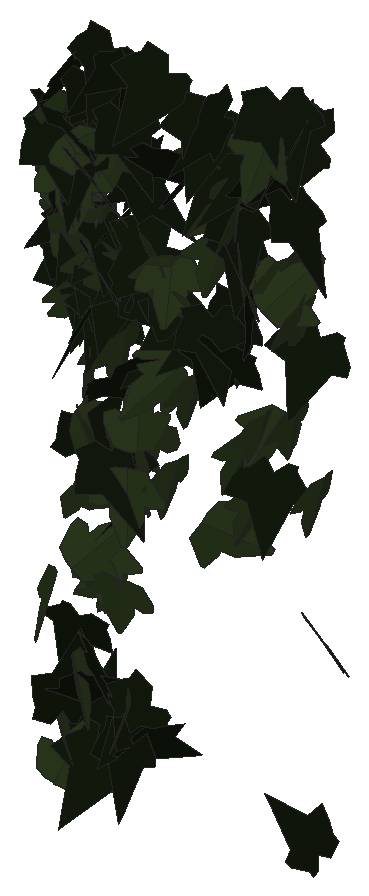
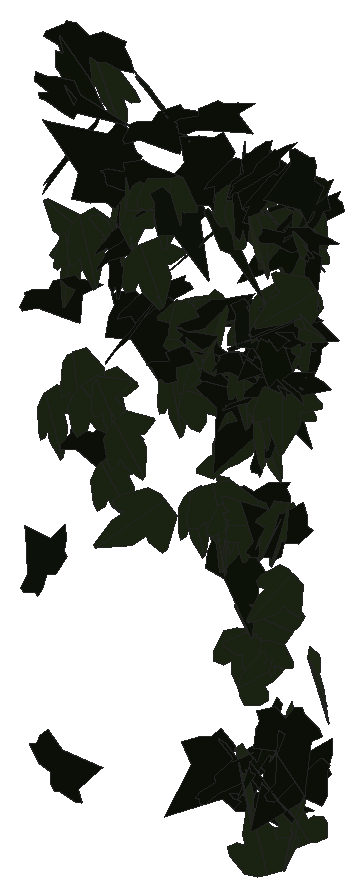
# SketchUp Ruby script. Lengths in inches.
U = 1.inch
M = Sketchup.active_model
def pt(a) = Geom::Point3d.new(a.map { |v| v * U })
def face(e, loops, mat)
  f = e.add_face(loops[0].map { |a| pt(a) })
  loops[1..].each { |l| e.add_face(l.map { |a| pt(a) }).erase! }
  f.material = f.back_material = mat if mat
  f
end
# faces: each face lists its corners as indices into pts; further lists are holes
def faces(e, pts, list, mat = nil) = list.each { |f| face(e, (f[0].is_a?(Array) ? f : [f]).map { |l| l.map { |i| pts[i] } }, mat) }
# xy, xz, yz: faces in a plane at the given z, y or x. An outline is a flat list of corners, or four numbers for a rectangle; further outlines are holes
def ring(l) = l.size == 4 ? [[l[0], l[1]], [l[2], l[1]], [l[2], l[3]], [l[0], l[3]]] : l.each_slice(2).to_a
def flat(e, list, mat, &to3) = list.each { |f| face(e, (f[0].is_a?(Array) ? f : [f]).map { |l| ring(l).map { |u, v| to3.(u, v) } }, mat) }
def xy(e, z, list, mat = nil) = flat(e, list, mat) { |x, y| [x, y, z] }
def xz(e, y, list, mat = nil) = flat(e, list, mat) { |x, z| [x, y, z] }
def yz(e, x, list, mat = nil) = flat(e, list, mat) { |y, z| [x, y, z] }
def lines(e, pts, list) = list.each { |a, b| e.add_line(pt(pts[a]), pt(pts[b])) }
# prism: a flat outline (further loops are holes) pulled along v
def prism(e, loops, v, mat = nil)
  f = face(e, loops, mat); d = Geom::Vector3d.new(v.map { |x| x * U })
  f.pushpull(f.normal.samedirection?(d) ? d.length : -d.length)
end
def box(e, o, s, mat = nil) = prism(e, [[o, [o[0] + s[0], o[1], o[2]], [o[0] + s[0], o[1] + s[1], o[2]], [o[0], o[1] + s[1], o[2]]]], [0, 0, s[2]], mat)
def at(x, y, z, deg = 0) = Geom::Transformation.translation(pt([x, y, z])) * Geom::Transformation.rotation(ORIGIN, Z_AXIS, deg.degrees)
def axes(o, x, y, z) = Geom::Transformation.new([*x, 0, *y, 0, *z, 0, *pt(o).to_a, 1])
def part(name) = M.definitions.add(name)
# library, detail: a bought-in or finely detailed component or shape, given as its bounding box
def library(name, o, s) = part(name).tap { |d| box(d.entities, o, s) }
def detail(e, o, s) = box(e.add_group.entities, o, s)
def put(e, d, t, mat = nil) = e.add_instance(d, t).tap { |i| i.material = mat if mat }
def group(e, t, mat = nil) = e.add_group.tap { |g| g.transformation = t; g.material = mat if mat }.entities
root = M.entities
M.materials.add("efeu1").color = [18, 25, 13]
M.materials.add("efeu2").color = [43, 57, 29]
c1 = part("ivyleaf_9")
p = [[1.54,2.16,1.25],[1.36,2.04,1.19],[-0.21,0.99,0.68],[-0.71,1.11,0.82],[-0.85,0.86,0.67],[-0.8,0.17,0.21],
  [-0.9,-0.01,0.1],[-0.67,-0.16,-0.02],[-0.08,-0.08,-0.05],[-0.03,-0.6,-0.4],[0.65,-0.88,-0.66],[0.83,-0.6,-0.49],
  [1.29,-0.42,-0.43],[1.8125,-0.07,-0.26],[1.21,0.44,0.15]]
faces(c1.entities,p,[[0,1,2,3,4,5,6,7,8,9,10,11,12,13,14]],"efeu1")
c2 = part("ivyleaf_10")
p = [[0,0.5,-0.03],[-0.0625,2.02,-0.43],[-0.19,2.01,-0.46],[-0.54,1.05,-0.29],[-0.52,0.625,-0.18],[-0.83,0.76,-0.28],
  [-1.16,0.64,-0.33],[-1.15,0.33,-0.24],[-0.77,-0.39,0.02],[-0.3,-0.51,0.16],[0.04,-0.48,0.23],[-0.02,2.01,-0.4375],
  [-0.06,2.01,-0.43],[0.04,-0.49,0.23],[0.67,-0.49,0.14],[1.38,0.36,-0.2],[1.375,0.51,-0.24],[0.81,0.65,-0.19],
  [0.62,0.59,-0.15],[0.6,1.09,-0.28],[0.5,1.23,-0.31]]
faces(c2.entities,p,[[0,1,2,3,4,5,6,7,8,9,10],[11,12,0,13,14,15,16,17,18,19,20]],"efeu2")
put(root,c1,axes([507.83,132.65,201.51],[0.08823,-0.14914,0.79199],[-0.21475,0.73614,0.17212],[-0.81009,-0.21139,0.04063]))
put(root,c1,axes([507.59,132.8,204.79],[-0.22478,0.50304,-0.56535],[-0.28414,0.47763,0.56442],[0.74774,0.33272,0.04453]))
put(root,c2,axes([507.55,132.72,188.94],[0.5578,-0.63656,0.09202],[0.06028,-0.06866,-0.85253],[0.69148,0.51949,0.00008]))
put(root,c1,axes([507.84,133.64,187.58],[0.3913,0.28613,-0.55356],[-0.43338,-0.35012,-0.47981],[-0.48799,0.54037,-0.01777]))
put(root,c2,axes([507.55,133.21,203.85],[0.11682,-0.66008,0.56389],[0.20973,-0.53066,-0.66464],[0.84243,0.22365,0.08727]))
put(root,c2,axes([508.34,133.24,200.28],[0.14149,0.1442,0.84892],[-0.89486,-0.00054,0.13841],[0.02527,-0.82671,0.14798]))
put(root,c1,axes([507.72,133.79,203.49],[-0.62241,-0.5033,-0.11717],[0.16276,-0.00276,-0.7889],[0.5327,-0.58721,0.10414]))
put(root,c2,axes([507.35,133.46,201.4],[0.29609,0.231,0.69601],[0.33312,0.60701,-0.34931],[-0.68825,0.39318,0.13036]))
put(root,c2,axes([507.83,133.82,198.22],[-0.40944,-0.70221,-0.07221],[0.04586,0.05597,-0.82985],[0.7607,-0.38133,0.01116]))
put(root,c1,axes([508.04,133.86,200.75],[-0.03628,-0.00307,-0.74142],[-0.02421,-0.71334,0.0043],[-0.76957,0.02259,0.03482]))
put(root,c2,axes([507.92,132.95,184.39],[-0.48542,0.61504,0.36711],[-0.21163,0.29393,-0.79211],[-0.73605,-0.49013,-0.01435]))
put(root,c1,axes([507.71,134.01,198.78],[-0.35915,-0.66076,-0.26235],[0.15194,0.21138,-0.76872],[0.74859,-0.35991,0.03016]))
put(root,c1,axes([508.11,134.05,199.85],[-0.44002,0.41627,-0.41612],[0.29026,-0.29669,-0.60563],[-0.55191,-0.48792,0.01325]))
put(root,c1,axes([507.94,132.85,185.15],[-0.29979,-0.38919,0.71445],[0.55362,0.46502,0.4894],[-0.64856,0.57684,0.08751]))
put(root,c1,axes([507.4375,133.03,204.11],[0.52831,-0.60031,0.08765],[0.16106,0.01421,-0.79498],[0.63457,0.49618,0.12881]))
put(root,c2,axes([507.87,133.06,199.88],[-0.73165,0.39673,-0.31358],[0.26626,-0.16665,-0.83209],[-0.42992,-0.77838,0.01832]))
put(root,c2,axes([508.18,133.49,197.84],[-0.61701,-0.45043,-0.12896],[0.10779,0.07369,-0.7566],[0.49291,-0.57994,0.00403]))
put(root,c1,axes([507.875,132.69,203.6],[0.05112,-0.8027,-0.32007],[-0.03615,0.30627,-0.83612],[0.92774,0.05617,-0.01494]))
put(root,c2,axes([508.23,133.42,193.97],[-0.59195,0.42254,0.1104],[-0.09381,0.06119,-0.71973],[-0.46107,-0.55492,0.0047]))
put(root,c1,axes([508.02,132.7,185.82],[0.6078,0.5937,0.15759],[0.10716,0.11474,-0.85074],[-0.65302,0.57142,0.00708]))
put(root,c2,axes([508.0625,133.46,191.89],[-0.28471,-0.36404,-0.5651],[0.33352,0.44715,-0.46738],[0.62267,-0.40596,-0.00804]))
put(root,c2,axes([508.21,133.37,194.08],[-0.04122,0.6181,0.34369],[-0.01625,0.33016,-0.64403],[-0.7568,-0.04075,-0.00489]))
put(root,c1,axes([508.43,133.56,200.625],[-0.65499,-0.43701,-0.09011],[0.07869,0.04708,-0.77741],[0.47468,-0.61082,0.00455]))
put(root,c1,axes([508.15,133.42,193.22],[-0.24418,-0.12481,0.67841],[0.63607,0.28081,0.26817],[-0.33152,0.6307,0.01486]))
put(root,c1,axes([507.96,133.28,199.95],[-0.14606,-0.25315,-0.77029],[0.35961,0.66163,-0.29841],[0.76504,-0.35933,-0.00679]))
put(root,c2,axes([508.1,132.52,183.33],[0.6501,0.27358,-0.33388],[0.31047,0.14327,0.68756],[0.33334,-0.66698,0.01075]))
put(root,c2,axes([507.84,132.91,200.04],[-0.00218,-0.10095,0.80218],[0.78223,0.28117,0.04024],[-0.30651,0.71826,0.097]))
put(root,c1,axes([508.48,133.75,199.83],[-0.53829,-0.51327,-0.22019],[0.22001,0.09562,-0.73983],[0.55782,-0.53302,0.07932]))
put(root,c2,axes([508.6,134.29,188.84],[-0.1192,0.12374,0.75106],[0.06288,-0.72653,0.13872],[0.78881,0.07662,0.10243]))
put(root,c1,axes([508.27,133.57,205],[0.36472,-0.6805,-0.43662],[-0.16234,0.4076,-0.77087],[0.79206,0.39689,0.04306]))
put(root,c1,axes([508.37,133.1,203.06],[-0.60944,-0.31216,-0.57338],[0.65229,-0.04204,-0.61816],[0.20668,-0.7878,0.26018]))
put(root,c1,axes([508.43,134.38,205.51],[-0.14976,-0.77891,0.2669],[-0.03446,-0.26512,-0.79303],[0.82265,-0.15291,0.01537]))
put(root,c1,axes([508.8,132.95,197.97],[-0.45384,0.48819,-0.44189],[0.29717,-0.32377,-0.6699],[-0.63265,-0.50229,0.00232]))
put(root,c1,axes([508.74,133.16,184.51],[-0.69852,0.44966,0.1023],[0.08168,-0.06353,0.81919],[0.49036,0.65112,0.00928]))
put(root,c1,axes([508.59,134.28,199.99],[-0.43553,-0.61017,0.31763],[0.03986,-0.39769,-0.70932],[0.68674,-0.36388,0.24261]))
put(root,c2,axes([508.6875,133.54,200.6875],[-0.02906,-0.81664,0.1158],[0.06027,-0.11295,-0.84755],[0.88809,-0.01905,0.06131]))
put(root,c2,axes([508.66,133.66,196.73],[0.25168,-0.80206,0.1969],[0.04548,-0.19207,-0.8405],[0.82462,0.25538,-0.01374]))
put(root,c2,axes([508.43,132.58,202.53],[0.87773,0.24491,0.12471],[0.12004,0.04671,-0.88267],[-0.26893,0.82019,0.01304]))
put(root,c1,axes([509.01,133.5625,200.31],[-0.36581,0.7294,-0.16348],[0.07341,-0.14174,-0.83637],[-0.80249,-0.34546,-0.00199]))
put(root,c2,axes([508.39,132.72,203.12],[0.33206,0.63205,0.41507],[0.20873,0.34965,-0.73074],[-0.77986,0.36271,-0.01885]))
put(root,c2,axes([508.75,133.92,203.34],[0.34835,-0.66525,0.07882],[0.0303,-0.07063,-0.76887],[0.72248,0.32372,-0.00577]))
put(root,c1,axes([508.875,133.74,198.85],[-0.79284,-0.23796,-0.24781],[0.26839,0.00287,-0.79921],[0.24545,-0.7718,0.07344]))
put(root,c1,axes([508.32,132.69,202.84],[0.84414,-0.26691,-0.04166],[-0.0398,0.01603,-0.85895],[0.28876,0.78247,0.00338]))
put(root,c2,axes([508.66,132.62,186.73],[-0.32703,0.74213,-0.16966],[0.06738,-0.15074,-0.83359],[-0.81787,-0.30916,-0.00084]))
put(root,c1,axes([508.39,133.95,196.16],[0.1022,-0.23603,0.65467],[0.22483,-0.59416,-0.26424],[0.69038,0.22844,-0.01086]))
put(root,c2,axes([508.72,133.58,182.75],[-0.56267,-0.52934,0.14175],[0.10232,0.09812,0.77253],[-0.53836,0.57189,-0.00134]))
put(root,c1,axes([508.71,133.04,186.95],[0.68181,-0.21049,-0.48764],[-0.45179,0.22105,-0.68895],[0.32249,0.75467,0.06579]))
put(root,c2,axes([508.62,133.79,189.76],[0.73936,0.30162,0.12368],[0.1156,0.052,-0.778],[-0.33052,0.69289,0.00455]))
put(root,c1,axes([508.93,134.1,205.1875],[-0.03426,-0.15436,-0.7374],[0.29574,-0.65979,0.13664],[-0.72576,-0.26157,0.09049]))
put(root,c2,axes([508.55,132.95,190.06],[0.37922,0.28564,-0.68694],[0.5192,0.4538,0.46987],[0.57835,-0.59468,0.0286]))
put(root,c2,axes([508.76,132.9375,196.57],[-0.15176,0.31577,-0.70998],[0.25853,-0.63961,-0.35892],[-0.7701,-0.27695,0.01942]))
put(root,c1,axes([508.96,133.86,197.78],[-0.39507,-0.66279,0.20863],[0.11374,-0.27748,-0.75373],[0.73918,-0.31154,0.22748]))
put(root,c2,axes([509.25,132.99,199.7],[-0.69264,-0.49041,0.01584],[-0.01025,-0.01266,-0.83963],[0.52979,-0.64139,0.00446]))
put(root,c1,axes([508.96,134.21,203.55],[0.03827,0.31837,0.73957],[-0.10903,-0.70398,0.33301],[0.83437,-0.1066,0.00959]))
put(root,c2,axes([509.07,134.43,203.58],[-0.05981,-0.18416,-0.78009],[0.0303,-0.752,0.18986],[-0.8336,-0.01412,0.06287]))
put(root,c1,axes([508.89,133.66,200.39],[0.00314,-0.7575,0.31667],[0.12135,-0.31277,-0.74936],[0.81201,0.04967,0.11077]))
put(root,c1,axes([509.44,132.95,184.17],[-0.78406,-0.43411,-0.05905],[0.10459,-0.05201,-0.87424],[0.46112,-0.72634,0.0979]))
put(root,c1,axes([509.27,133.72,199.02],[-0.40992,-0.71059,-0.07124],[0.03052,0.06257,-0.83781],[0.77039,-0.38058,-0.00472]))
put(root,c1,axes([508.9,133.125,199.51],[0.1803,-0.46852,0.59657],[0.30705,-0.50244,-0.51284],[0.73862,0.32323,0.06756]))
put(root,c2,axes([509.63,133.26,189.32],[-0.81636,-0.16825,0.13142],[-0.13501,-0.01997,-0.80533],[0.1828,-0.76612,-0.00786]))
put(root,c2,axes([509.02,134,193.7],[-0.31907,0.09238,-0.68974],[0.67749,-0.21538,-0.32182],[-0.25296,-0.69335,0.00807]))
put(root,c1,axes([509.98,133.21,192.07],[-0.18307,0.81913,0.11633],[-0.06771,0.10111,-0.86892],[-0.8903,-0.17613,0.04217]))
put(root,c2,axes([509.87,133.15,203.66],[-0.61061,-0.49609,0.29463],[-0.13166,-0.28464,-0.77138],[0.60278,-0.5647,0.12998]))
put(root,c2,axes([509.76,133.25,185.375],[0.38954,-0.72474,-0.22287],[-0.10474,0.19111,-0.84192],[0.80948,0.3735,-0.00168]))
put(root,c2,axes([509.76,133.625,193.54],[-0.298,-0.65377,-0.27245],[0.09754,0.24619,-0.7379],[0.75437,-0.29009,-0.01222]))
put(root,c1,axes([510.3,133.55,202.77],[-0.63559,0.57987,0.01524],[-0.00774,0.0136,-0.85922],[-0.62641,-0.58853,-0.00485]))
put(root,c1,axes([509.86,134.2,185.18],[-0.31636,-0.65996,0.4688],[-0.15844,-0.44311,-0.73072],[0.79386,-0.35144,0.04098]))
put(root,c2,axes([510.16,133.97,194.12],[-0.54499,-0.57299,0.19263],[-0.14405,-0.1293,-0.79392],[0.6342,-0.52176,-0.0148]))
put(root,c2,axes([510.39,133.44,192.89],[0.22135,-0.25303,-0.772],[-0.37051,0.66101,-0.33284],[0.76165,0.39509,0.06245]))
put(root,c2,axes([510.2,132.62,197.71],[-0.02838,-0.79904,-0.10378],[0.01308,0.09944,-0.83141],[0.86957,-0.02757,0.00912]))
put(root,c1,axes([509.82,132.7,193.87],[-0.06217,-0.68762,-0.4716],[0.13956,0.4414,-0.71316],[0.87856,-0.11878,0.07992]))
put(root,c2,axes([510.13,133.84,200.14],[-0.64876,0.52729,-0.06568],[0.06479,-0.02737,-0.83104],[-0.56987,-0.60339,-0.0197]))
put(root,c1,axes([510.43,134.16,200.04],[-0.588,-0.55261,0.41769],[-0.22986,-0.36119,-0.80143],[0.65346,-0.6243,0.09394]))
put(root,c1,axes([510.27,132.17,196.76],[0.44264,0.75566,0.14859],[0.07247,0.12614,-0.89404],[-0.82741,0.41531,0.00118]))
put(root,c1,axes([510.04,132.92,204.64],[0.17079,-0.72936,-0.33278],[-0.05623,0.31606,-0.77601],[0.85834,0.16583,0.01538]))
put(root,c2,axes([510.15,133.3,193.7],[-0.46374,0.44987,-0.53081],[0.3234,-0.41698,-0.64423],[-0.65979,-0.52058,0.05732]))
put(root,c1,axes([511.09,133.92,198.71],[-0.67589,0.05553,0.47685],[-0.49661,-0.0025,-0.65241],[-0.04678,-0.77581,0.03623]))
put(root,c1,axes([510.38,132.72,185.08],[-0.64206,-0.16828,-0.52487],[0.53327,0.10716,-0.64208],[0.21386,-0.77243,0.02527]))
put(root,c2,axes([510.375,132.55,193.21],[0.90829,0.18172,0.09552],[0.07894,0.09489,-0.89126],[-0.20524,0.84068,0.07995]))
put(root,c2,axes([510.58,132.78,194.78],[0.27542,0.7945,-0.22775],[0.06243,0.21142,0.86774],[0.88786,-0.26132,0.00963]))
put(root,c1,axes([510.4,133.13,202.71],[0.55852,-0.49494,-0.37368],[-0.09262,0.4072,-0.71173],[0.65401,0.48034,0.21832]))
put(root,c2,axes([510.97,133.78,199.82],[-0.47581,-0.64235,0.05975],[-0.03497,-0.04746,-0.81008],[0.69563,-0.44176,0.00015]))
put(root,c1,axes([510.61,132.83,184.86],[0.50567,0.51382,0.36711],[0.25703,0.26212,-0.72091],[-0.57682,0.56724,0.00059]))
put(root,c1,axes([511.03,133.5,206.02],[-0.55005,-0.61416,0.19272],[-0.0722,-0.19304,-0.82123],[0.63963,-0.54994,0.07304]))
put(root,c2,axes([511.08,133.75,198.76],[-0.82182,0.16308,-0.06054],[0.06095,-0.01447,-0.80935],[-0.1768,-0.76303,0.00241]))
put(root,c2,axes([511.16,133.72,193.42],[-0.01132,-0.77015,0.09847],[0.01978,-0.09873,-0.76995],[0.77617,-0.00872,0.02105]))
put(root,c2,axes([511.375,133.23,196.72],[-0.2836,-0.31519,0.76725],[-0.07796,-0.79714,-0.35629],[0.8258,-0.1835,0.22986]))
put(root,c2,axes([511.11,133.63,199.78],[0.65305,0.4741,-0.03684],[-0.02976,-0.02171,-0.807],[-0.47459,0.65373,-0.00008]))
put(root,c1,axes([511.6,134.04,198.06],[-0.77715,-0.42242,0.22217],[-0.19155,-0.11279,-0.88451],[0.43716,-0.80038,0.00739]))
put(root,c1,axes([511.8,133.7,203.07],[-0.36266,0.72173,-0.17639],[0.02859,-0.18258,-0.80584],[-0.74242,-0.35958,0.05514]))
put(root,c1,axes([511.04,132.53,203.82],[0.81239,0.16006,0.30836],[0.30444,0.09839,-0.79899],[-0.19935,0.80253,0.03645]))
put(root,c2,axes([512.03,133.8,203.4],[-0.81131,-0.01771,0.15561],[-0.15582,0.00872,-0.81141],[0.01575,-0.82605,-0.0119]))
put(root,c2,axes([512.26,133.24,196.83],[-0.00653,-0.79512,0.00393],[0.00014,-0.00393,-0.79515],[0.79513,-0.00653,0.00017]))
put(root,c2,axes([512.68,133.97,201.02],[-0.3094,-0.71411,0.24873],[-0.01999,-0.26093,-0.774],[0.75593,-0.29919,0.08134]))
put(root,c1,axes([512.72,133.52,205.24],[-0.39699,-0.73355,-0.0254],[0.01047,0.02322,-0.83408],[0.73391,-0.39713,-0.00184]))
put(root,c2,axes([512.94,134.09,202.6],[0.02675,0.33963,-0.7723],[-0.31646,-0.71223,-0.32418],[-0.78208,0.29981,0.10476]))
put(root,c1,axes([513.19,134.12,203.6875],[-0.75234,-0.42413,0.04435],[-0.03886,-0.02137,-0.86366],[0.42467,-0.75335,-0.00047]))
put(root,c1,axes([512.87,134.43,198.79],[0.13175,-0.76568,0.26519],[0.02058,-0.26543,-0.77658],[0.81004,0.13127,-0.0234]))
put(root,c1,axes([513.54,132.89,205.82],[-0.78243,0.25969,-0.15704],[0.13375,-0.09474,-0.82306],[-0.27242,-0.79239,0.04694]))
put(root,c2,axes([513.01,133.29,192.45],[-0.34145,-0.38676,-0.75955],[0.62672,0.44065,-0.50611],[0.5777,-0.70664,0.10012]))
put(root,c1,axes([513.125,134.21,202.03],[0.06107,-0.80177,-0.0838],[0.00313,0.08428,-0.80404],[0.80613,0.06041,0.00947]))
put(root,c2,axes([513.57,133.45,202.6875],[0.24249,-0.75581,-0.43029],[-0.1194,0.41354,-0.79368],[0.86148,0.27006,0.01111]))
put(root,c1,axes([513.18,132.93,199.23],[-0.02686,-0.77697,-0.22063],[0.02167,0.21998,-0.77732],[0.8074,-0.03175,0.01353]))
put(root,c2,axes([513.61,133.9,195],[-0.0726,-0.73083,0.2927],[-0.04651,-0.28945,-0.73424],[0.78589,-0.08465,-0.01641]))
put(root,c1,axes([513.74,132.59,198.54],[0.43068,0.40867,-0.6231],[-0.43019,-0.45128,-0.59332],[-0.60844,0.60834,-0.02156]))
put(root,c1,axes([513.4,134.08,201.375],[-0.01396,-0.78957,0.17307],[-0.01456,-0.17282,-0.78961],[0.80818,-0.01675,-0.01123]))
put(root,c2,axes([514.07,133.9,193.51],[-0.10366,-0.72072,0.30819],[-0.05782,-0.30299,-0.72802],[0.78171,-0.11798,-0.01298]))
put(root,c2,axes([514.39,133.54,196.1],[-0.0241,-0.79406,-0.01036],[0.00004,0.01036,-0.79442],[0.79412,-0.0241,-0.00028]))
put(root,c2,axes([514.55,134.12,195.9],[-0.34451,-0.57467,0.50948],[-0.09383,-0.52271,-0.65304],[0.76224,-0.32407,0.14988]))
put(root,c2,axes([514.86,132.26,201.32],[-0.51504,0.32118,0.63002],[-0.52892,0.34237,-0.60694],[-0.46939,-0.73823,-0.00738]))
put(root,c1,axes([514.01,133.55,203.26],[0.40415,0.73771,-0.2474],[0.12219,0.21515,0.84115],[0.76843,-0.4222,-0.00363]))
put(root,c1,axes([514.37,133.2,199.5],[0.0339,0.2424,0.91267],[-0.0624,-0.91069,0.24419],[0.94225,-0.06903,-0.01667]))
put(root,c1,axes([514.73,133.69,194.51],[-0.3935,-0.6556,-0.22542],[0.12156,0.18994,-0.7646],[0.68253,-0.4118,0.00622]))
put(root,c2,axes([514.9375,133.9,201.1],[-0.01243,-0.86291,0.05121],[-0.00298,-0.05118,-0.86299],[0.86442,-0.01258,-0.00224]))
put(root,c2,axes([515.1,132.79,205.62],[0.93061,-0.20864,-0.13188],[-0.12654,0.03838,-0.95366],[0.21192,0.93912,0.00968]))
put(root,c2,axes([515.3,133.84,196.54],[0.00744,-0.79412,-0.10304],[-0.00476,0.103,-0.79414],[0.80076,0.00799,-0.00376]))
put(root,c1,axes([515.95,134.1,205.32],[-0.66283,0.12822,0.51203],[-0.51133,0.048,-0.67394],[-0.13099,-0.83619,0.03983]))
put(root,c2,axes([515.12,133.3,200.42],[0.64633,0.15459,-0.64452],[0.60619,0.22614,0.66214],[0.26801,-0.88431,0.05666]))
put(root,c2,axes([515.75,133.47,200.13],[-0.01304,-0.75711,-0.35889],[0.00146,0.35891,-0.75721],[0.83786,-0.01241,-0.00427]))
put(root,c1,axes([516.24,133.69,183.0625],[-0.08252,0.05785,0.78716],[-0.62122,0.48346,-0.10065],[-0.48688,-0.62665,-0.00499]))
put(root,c1,axes([515.44,133.09,206.82],[-0.46588,-0.49417,-0.62927],[0.46219,0.42817,-0.67843],[0.65311,-0.65551,0.03124]))
put(root,c1,axes([515.96,133.47,206.22],[-0.58617,0.35221,-0.49475],[0.38289,-0.31941,-0.68103],[-0.47141,-0.69739,0.06205]))
put(root,c1,axes([515.9,134.24,198.98],[-0.44541,-0.69657,-0.01807],[0.00618,0.01749,-0.82679],[0.69678,-0.44543,-0.00422]))
put(root,c1,axes([515.56,133.53,203.48],[0.40719,-0.80713,-0.17965],[-0.08403,0.15883,-0.90402],[0.8226,0.41576,-0.00341]))
put(root,c2,axes([516.43,133.58,194.75],[0.0786,-0.7876,0.0599],[0.0107,-0.05913,-0.7915],[0.78981,0.07918,0.00477]))
put(root,c1,axes([516.25,134,189.64],[0.10854,-0.43292,0.64366],[0.38344,-0.53502,-0.42452],[0.6743,0.37393,0.13779]))
